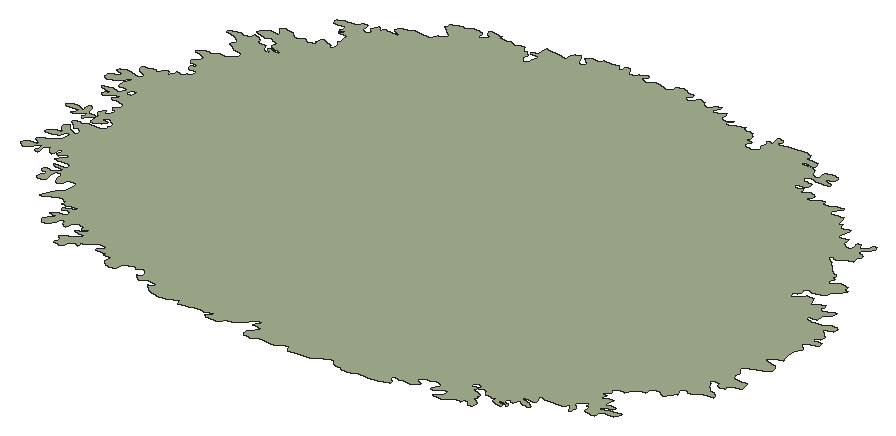
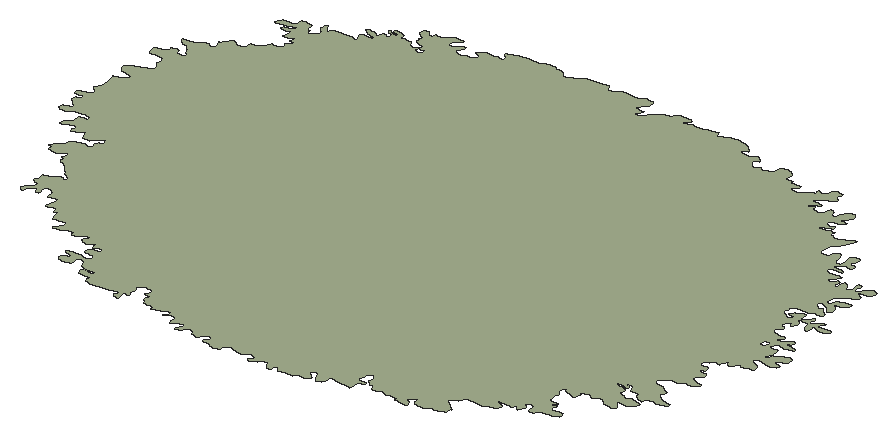
# SketchUp Ruby script. Lengths in inches.
U = 1.inch
M = Sketchup.active_model
def pt(a) = Geom::Point3d.new(a.map { |v| v * U })
def face(e, loops, mat)
  f = e.add_face(loops[0].map { |a| pt(a) })
  loops[1..].each { |l| e.add_face(l.map { |a| pt(a) }).erase! }
  f.material = f.back_material = mat if mat
  f
end
# faces: each face lists its corners as indices into pts; further lists are holes
def faces(e, pts, list, mat = nil) = list.each { |f| face(e, (f[0].is_a?(Array) ? f : [f]).map { |l| l.map { |i| pts[i] } }, mat) }
# xy, xz, yz: faces in a plane at the given z, y or x. An outline is a flat list of corners, or four numbers for a rectangle; further outlines are holes
def ring(l) = l.size == 4 ? [[l[0], l[1]], [l[2], l[1]], [l[2], l[3]], [l[0], l[3]]] : l.each_slice(2).to_a
def flat(e, list, mat, &to3) = list.each { |f| face(e, (f[0].is_a?(Array) ? f : [f]).map { |l| ring(l).map { |u, v| to3.(u, v) } }, mat) }
def xy(e, z, list, mat = nil) = flat(e, list, mat) { |x, y| [x, y, z] }
def xz(e, y, list, mat = nil) = flat(e, list, mat) { |x, z| [x, y, z] }
def yz(e, x, list, mat = nil) = flat(e, list, mat) { |y, z| [x, y, z] }
def lines(e, pts, list) = list.each { |a, b| e.add_line(pt(pts[a]), pt(pts[b])) }
# prism: a flat outline (further loops are holes) pulled along v
def prism(e, loops, v, mat = nil)
  f = face(e, loops, mat); d = Geom::Vector3d.new(v.map { |x| x * U })
  f.pushpull(f.normal.samedirection?(d) ? d.length : -d.length)
end
def box(e, o, s, mat = nil) = prism(e, [[o, [o[0] + s[0], o[1], o[2]], [o[0] + s[0], o[1] + s[1], o[2]], [o[0], o[1] + s[1], o[2]]]], [0, 0, s[2]], mat)
def at(x, y, z, deg = 0) = Geom::Transformation.translation(pt([x, y, z])) * Geom::Transformation.rotation(ORIGIN, Z_AXIS, deg.degrees)
def axes(o, x, y, z) = Geom::Transformation.new([*x, 0, *y, 0, *z, 0, *pt(o).to_a, 1])
def part(name) = M.definitions.add(name)
# library, detail: a bought-in or finely detailed component or shape, given as its bounding box
def library(name, o, s) = part(name).tap { |d| box(d.entities, o, s) }
def detail(e, o, s) = box(e.add_group.entities, o, s)
def put(e, d, t, mat = nil) = e.add_instance(d, t).tap { |i| i.material = mat if mat }
def group(e, t, mat = nil) = e.add_group.tap { |g| g.transformation = t; g.material = mat if mat }.entities
root = M.entities
M.materials.add("Boxwoodplan").color = [166, 177, 144]
xy(root,9.058,[[[105.479,67.129,105.368,67.133,105.273,67.159,105.217,67.215,105.216,67.317,105.242,67.382,105.305,67.445,105.354,67.509,105.413,67.606,105.226,67.635,105.136,67.644,105.156,67.732,105.242,67.79,105.273,67.8,105.268,67.846,105.179,67.877,105.063,67.837,104.966,67.706,104.824,67.551,104.663,67.464,104.557,67.441,104.497,67.416,104.481,67.373,104.336,67.281,104.143,67.251,104.054,67.26,103.973,67.306,103.973,67.328,104.019,67.359,104.109,67.437,104.178,67.483,104.088,67.498,103.976,67.48,103.856,67.436,103.662,67.454,103.565,67.447,103.439,67.403,103.238,67.356,103.149,67.349,103.111,67.443,103.103,67.465,103.036,67.473,102.947,67.454,102.779,67.336,102.579,67.328,102.349,67.353,102.182,67.446,102.04,67.61,102.223,67.702,102.124,67.756,101.988,67.772,101.862,67.749,101.789,67.697,101.709,67.672,101.593,67.738,101.551,67.806,101.638,67.847,101.665,67.907,101.67,67.957,101.629,68.009,101.556,68.085,101.471,68.117,101.384,68.064,101.317,68.038,101.261,68.08,101.245,68.103,101.221,68.121,101.191,68.111,101.112,68.058,101.04,68.01,100.964,67.923,100.953,67.79,100.881,67.749,100.831,67.723,100.771,67.725,100.672,67.746,100.586,67.793,100.542,67.861,100.533,67.951,100.542,68.018,100.555,68.04,100.536,68.08,100.323,68.1,100.391,68.135,100.364,68.136,100.272,68.13,100.102,68.146,100.025,68.173,100.008,68.206,100.022,68.224,100.148,68.314,100.145,68.371,100.061,68.393,99.901,68.39,99.771,68.319,99.673,68.233,99.599,68.199,99.551,68.172,99.55,68.154,99.587,68.101,99.571,68.046,99.5,68.081,99.437,68.121,99.376,68.072,99.353,68.017,99.322,67.904,99.274,67.855,99.201,67.822,99.11,67.816,99.04,67.841,99.022,67.874,99.029,67.892,99.05,67.932,99.072,67.991,99.041,68.048,98.94,68.149,99.054,68.229,99.115,68.269,99.194,68.285,99.262,68.315,99.317,68.37,99.401,68.476,99.33,68.503,99.25,68.511,99.118,68.53,99.079,68.565,99.087,68.584,99.161,68.62,99.323,68.657,99.366,68.709,99.361,68.748,99.335,68.764,99.185,68.711,99.139,68.732,99.14,68.752,99.162,68.814,99.001,68.825,98.921,68.833,98.867,68.826,98.859,68.806,98.843,68.71,98.828,68.642,98.787,68.591,98.74,68.578,98.72,68.594,98.661,68.639,98.617,68.757,98.577,68.783,98.55,68.784,98.497,68.777,98.49,68.757,98.488,68.641,98.433,68.523,98.373,68.449,98.293,68.419,98.214,68.422,98.167,68.448,98.134,68.506,98.135,68.564,98.188,68.677,98.302,68.784,98.323,68.803,98.309,68.823,98.283,68.829,98.202,68.847,98.122,68.86,98.095,68.875,98.101,68.895,98.122,68.914,98.27,68.982,98.432,69.005,98.474,69.108,98.448,69.169,98.401,69.191,98.373,69.187,98.21,69.168,98.17,69.2,98.176,69.22,98.204,69.279,98.361,69.334,98.533,69.403,98.582,69.442,98.568,69.463,98.472,69.436,98.3,69.417,98.156,69.372,98.067,69.386,98.04,69.392,98.047,69.412,98.067,69.426,98.122,69.47,98.095,69.507,98.067,69.503,97.985,69.511,97.93,69.56,97.916,69.601,97.888,69.597,97.806,69.575,97.649,69.489,97.499,69.413,97.425,69.38,97.37,69.392,97.383,69.412,97.403,69.452,97.429,69.469,97.454,69.55,97.503,69.65,97.535,69.759,97.586,69.812,97.66,69.852,97.704,69.972,97.726,70.112,97.745,70.227,97.741,70.285,97.696,70.321,97.616,70.335,97.529,70.335,97.456,70.31,97.446,70.245,97.446,70.184,97.413,70.124,97.325,70.087,97.269,70.096,97.23,70.155,97.22,70.216,97.194,70.337,97.188,70.4,97.148,70.453,97.12,70.475,97.083,70.491,97.024,70.479,96.989,70.46,96.988,70.428,96.98,70.366,96.982,70.229,97.007,70.167,96.999,70.103,96.949,70.038,96.9,70.01,96.862,69.998,96.825,70.003,96.783,70.011,96.765,70.039,96.761,70.166,96.782,70.223,96.827,70.276,96.843,70.306,96.834,70.334,96.777,70.34,96.696,70.346,96.658,70.362,96.635,70.39,96.632,70.453,96.648,70.483,96.682,70.499,96.855,70.472,96.933,70.497,96.983,70.526,97.043,70.573,97.057,70.636,97.034,70.662,96.99,70.664,96.912,70.67,96.82,70.681,96.719,70.717,96.701,70.746,96.706,70.76,96.726,70.763,96.785,70.775,96.961,70.761,97.05,70.787,97.063,70.844,97.037,70.907,96.965,70.946,96.886,70.953,96.772,70.946,96.673,70.921,96.589,70.939,96.585,70.968,96.606,70.997,96.652,71.054,96.719,71.11,96.772,71.19,96.763,71.224,96.719,71.241,96.654,71.24,96.536,71.14,96.496,71.141,96.462,71.161,96.483,71.22,96.5,71.287,96.456,71.35,96.416,71.366,96.396,71.367,96.391,71.352,96.395,71.306,96.392,71.164,96.351,71.102,96.311,71.108,96.277,71.131,96.179,71.262,96.154,71.327,96.13,71.355,96.114,71.344,96.059,71.293,96.024,71.234,96.043,71.103,96.048,71.037,96.028,70.971,95.979,70.962,95.944,70.978,95.934,71.023,95.954,71.155,95.964,71.233,95.964,71.27,95.949,71.282,95.934,71.272,95.854,71.237,95.815,71.183,95.805,71.12,95.766,71.077,95.629,70.987,95.59,70.977,95.545,70.986,95.466,71.026,95.445,71.056,95.449,71.089,95.482,71.151,95.58,71.237,95.669,71.263,95.759,71.263,95.854,71.267,95.794,71.318,95.642,71.404,95.626,71.466,95.679,71.503,95.77,71.573,95.889,71.635,96.008,71.709,96.043,71.723,96.069,71.746,96.096,71.789,96.099,71.882,96.131,72.003,96.132,72.065,96.111,72.086,96.09,72.095,96.027,72.109,95.993,72.104,95.99,72.088,96.001,71.996,95.96,71.934,95.912,71.899,95.834,71.871,95.763,71.858,95.603,71.833,95.568,71.839,95.554,71.853,95.555,71.86,95.563,71.901,95.58,71.947,95.622,71.995,95.692,72.042,95.75,72.063,95.809,72.065,95.847,72.068,95.867,72.075,95.89,72.096,95.886,72.121,95.831,72.151,95.763,72.207,95.731,72.264,95.727,72.331,95.74,72.382,95.793,72.426,95.819,72.432,95.83,72.425,95.849,72.411,95.892,72.35,95.941,72.304,96.07,72.226,96.143,72.192,96.179,72.177,96.199,72.184,96.223,72.206,96.229,72.222,96.241,72.263,96.225,72.32,96.183,72.366,96.15,72.389,96.117,72.401,96.057,72.401,95.983,72.404,95.939,72.446,95.853,72.519,95.795,72.569,95.756,72.617,95.756,72.646,95.78,72.671,95.837,72.698,95.872,72.703,95.913,72.7,95.973,72.679,96.034,72.677,96.07,72.684,96.105,72.726,96.153,72.757,96.213,72.764,96.284,72.764,96.4375,72.771,96.578,72.792,96.61,72.808,96.611,72.826,96.605,72.868,96.594,72.913,96.605,72.957,96.635,73.06,96.621,73.083,96.599,73.097,96.542,73.126,96.488,73.164,96.416,73.192,96.343,73.195,96.292,73.184,96.271,73.17,96.246,73.119,96.251,73.098,96.263,73.093,96.286,73.088,96.437,73.076,96.463,73.071,96.469,73.0625,96.459,73.046,96.42,73.007,96.374,72.964,96.31,72.928,96.248,72.884,96.175,72.849,96.138,72.852,96.119,72.863,96.093,72.9,96.086,72.995,96.069,73.02,96.087,73.034,96.094,73.077,96.088,73.088,96.076,73.088,96.062,73.087,96.036,73.083,96.003,73.076,95.986,73.065,95.905,72.97,95.873,72.915,95.842,72.892,95.819,72.895,95.793,72.916,95.784,72.932,95.778,72.973,95.806,73.057,95.812,73.102,95.803,73.13,95.782,73.137,95.744,73.128,95.724,73.114,95.678,73.064,95.557,72.957,95.52,72.932,95.495,72.927,95.457,72.935,95.445,72.951,95.537,73.057,95.599,73.102,95.613,73.129,95.613,73.145,95.604,73.152,95.592,73.148,95.578,73.143,95.546,73.131,95.463,73.108,95.295,73.089,95.222,73.096,95.175,73.121,95.153,73.149,95.152,73.165,95.169,73.217,95.216,73.264,95.277,73.281,95.347,73.284,95.422,73.266,95.549,73.223,95.635,73.197,95.647,73.201,95.647,73.209,95.646,73.22,95.637,73.239,95.613,73.287,95.611,73.342,95.619,73.407,95.63,73.437,95.648,73.45,95.696,73.413,95.736,73.363,95.763,73.317,95.772,73.255,95.785,73.204,95.799,73.176,95.823,73.175,95.957,73.157,96.03,73.144,96.065,73.14,96.083,73.154,96.099,73.202,96.043,73.244,95.985,73.309,95.967,73.335,95.967,73.352,96.001,73.46,96.031,73.483,96.059,73.489,96.073,73.477,96.082,73.459,96.111,73.414,96.123,73.39,96.135,73.391,96.156,73.404,96.236,73.482,96.252,73.528,96.254,73.579,96.24,73.611,96.219,73.623,96.155,73.646,96.116,73.666,96.107,73.687,96.123,73.736,96.179,73.773,96.214,73.795,96.227,73.816,96.234,73.869,96.233,73.916,96.137,73.992,95.994,74.014,95.931,74.031,95.897,74.013,95.868,74.014,95.799,74.031,95.78,74.058,95.79,74.082,95.916,74.185,95.909,74.217,95.887,74.233,95.843,74.225,95.814,74.216,95.688,74.154,95.648,74.107,95.598,74.063,95.529,74.049,95.501,74.05,95.454,74.102,95.482,74.126,95.5,74.165,95.532,74.188,95.625,74.22,95.67,74.25,95.66,74.281,95.647,74.283,95.637,74.276,95.611,74.27,95.571,74.273,95.436,74.284,95.29,74.3125,95.266,74.327,95.271,74.347,95.296,74.375,95.509,74.435,95.573,74.434,95.633,74.419,95.694,74.391,95.72,74.393,95.727,74.403,95.776,74.48,95.799,74.495,95.806,74.515,95.805,74.557,95.805,74.583,95.795,74.593,95.781,74.591,95.724,74.591,95.666,74.585,95.619,74.568,95.595,74.576,95.575,74.596,95.55,74.63,95.53,74.718,95.54,74.806,95.57,74.848,95.576,74.88,95.589,74.923,95.627,74.944,95.622,74.99,95.6,75.026,95.511,75.003,95.494,74.969,95.495,74.95,95.498,74.886,95.417,74.839,95.276,74.745,95.121,74.7,95.037,74.725,94.995,74.778,94.985,74.904,95.114,74.99,95.196,75.003,95.24,75.027,95.264,75.061,95.262,75.081,95.177,75.112,95.104,75.138,95.042,75.194,95.077,75.249,95.153,75.278,95.249,75.312,95.314,75.311,95.492,75.267,95.585,75.246,95.669,75.25,95.72,75.269,95.726,75.289,95.711,75.355,95.65,75.407,95.605,75.415,95.493,75.485,95.446,75.527,95.431,75.564,95.425,75.617,95.425,75.644,95.4375,75.659,95.48,75.695,95.531,75.709,95.645,75.741,95.675,75.751,95.716,75.75,95.766,75.746,95.778,75.733,95.793,75.703,95.808,75.689,95.817,75.689,95.846,75.692,95.862,75.704,95.882,75.754,95.91,75.787,95.927,75.81,95.929,75.835,95.946,75.86,95.965,75.872,96.013,75.884,96.052,75.877,96.074,75.833,96.078,75.781,96.094,75.755,96.116,75.754,96.157,75.796,96.182,75.838,96.197,75.942,96.212,75.968,96.245,75.975,96.276,75.974,96.296,75.963,96.317,75.94,96.349,75.94,96.401,75.961,96.446,76.007,96.46,76.032,96.449,76.046,96.509,76.043,96.538,76.046,96.553,76.066,96.558,76.114,96.592,76.155,96.627,76.2,96.573,76.243,96.505,76.272,96.468,76.271,96.436,76.261,96.393,76.249,96.352,76.255,96.33,76.271,96.308,76.295,96.285,76.397,96.298,76.423,96.304,76.439,96.314,76.443,96.418,76.463,96.464,76.472,96.483,76.483,96.473,76.486,96.387,76.514,96.321,76.526,96.293,76.519,96.257,76.52,96.221,76.52,96.186,76.532,96.147,76.582,96.129,76.611,96.129,76.642,96.145,76.663,96.174,76.678,96.205,76.697,96.213,76.725,96.243,76.782,96.27,76.836,96.276,76.89,96.268,76.917,96.228,76.928,96.15,76.954,95.977,77.001,95.942,77.018,95.925,77.042,95.96,77.097,96.005,77.131,96.05,77.159,96.105,77.178,96.158,77.1875,96.21,77.184,96.265,77.16,96.321,77.162,96.347,77.167,96.361,77.187,96.378,77.228,96.415,77.264,96.435,77.282,96.462,77.284,96.531,77.267,96.593,77.256,96.619,77.253,96.643,77.268,96.729,77.336,96.817,77.401,96.87,77.498,96.867,77.542,96.825,77.579,96.708,77.617,96.583,77.647,96.496,77.719,96.439,77.755,96.37,77.776,96.342,77.788,96.329,77.808,96.351,77.855,96.399,77.896,96.397,77.981,96.347,78.06,96.217,78.116,95.977,78.196,95.928,78.212,95.908,78.246,95.979,78.31,96.1,78.362,96.206,78.367,96.263,78.353,96.307,78.327,96.355,78.317,96.408,78.326,96.469,78.337,96.499,78.368,96.513,78.448,96.531,78.483,96.584,78.482,96.641,78.471,96.689,78.451,96.756,78.392,96.781,78.358,96.795,78.318,96.796,78.249,96.802,78.245,96.81,78.249,96.837,78.262,96.889,78.268,96.977,78.271,97.057,78.235,97.092,78.17,97.116,78.092,97.186,78.047,97.227,78.035,97.244,78.034,97.271,78.043,97.367,78.05,97.383,78.055,97.363,78.071,97.3,78.095,97.249,78.099,97.21,78.118,97.191,78.152,97.188,78.164,97.192,78.184,97.207,78.191,97.241,78.192,97.283,78.185,97.39,78.156,97.504,78.152,97.556,78.159,97.575,78.162,97.601,78.173,97.557,78.203,97.515,78.213,97.429,78.228,97.371,78.242,97.331,78.244,97.308,78.248,97.283,78.263,97.232,78.289,97.185,78.315,97.162,78.348,97.173,78.404,97.201,78.442,97.242,78.471,97.202,78.502,97.147,78.517,97.105,78.52,97.049,78.528,97.018,78.555,97.001,78.591,96.986,78.6,96.958,78.599,96.842,78.571,96.79,78.557,96.74,78.559,96.693,78.562,96.643,78.578,96.595,78.595,96.555,78.602,96.469,78.65,96.495,78.662,96.496,78.669,96.508,78.709,96.523,78.745,96.549,78.782,96.58,78.814,96.624,78.839,96.677,78.862,96.723,78.873,96.829,78.867,96.906,78.862,96.939,78.858,96.949,78.857,96.949,78.87,96.941,78.912,96.92,78.956,96.884,78.995,96.842,79.026,96.809,79.073,96.811,79.096,96.821,79.117,96.869,79.147,96.921,79.17,96.947,79.169,96.973,79.163,97.028,79.148,97.095,79.142,97.143,79.127,97.166,79.114,97.185,79.095,97.228,79.055,97.267,79.02,97.312,78.989,97.369,78.976,97.422,78.981,97.468,79.01,97.499,79.046,97.548,79.084,97.574,79.083,97.597,79.069,97.637,79.027,97.684,78.994,97.8125,79.019,97.887,79.037,97.928,79.065,97.934,79.085,97.912,79.102,97.861,79.124,97.852,79.147,97.86,79.169,97.875,79.214,97.882,79.273,97.886,79.299,97.909,79.315,97.937,79.316,97.967,79.308,98.009,79.288,98.143,79.248,98.203,79.226,98.243,79.193,98.269,79.153,98.284,79.13,98.291,79.123,98.301,79.126,98.309,79.131,98.341,79.176,98.347,79.212,98.337,79.315,98.316,79.362,98.292,79.397,98.256,79.436,98.246,79.466,98.258,79.477,98.269,79.475,98.29,79.476,98.29,79.484,98.295,79.508,98.287,79.549,98.273,79.705,98.275,79.782,98.159,79.802,98.062,79.804,98,79.8125,97.982,79.819,97.968,79.83,97.981,79.839,98.094,79.882,98.128,79.911,98.128,79.924,98.105,79.948,98.069,79.952,98.016,79.94,97.968,79.918,97.95,79.919,97.935,79.945,97.962,80.028,97.964,80.069,97.964,80.082,97.94,80.103,97.851,80.085,97.738,80.088,97.628,80.105,97.567,80.185,97.565,80.213,97.603,80.25,97.7,80.303,97.748,80.33,97.803,80.335,97.927,80.332,98.019,80.337,98.078,80.346,98.118,80.384,98.159,80.418,98.166,80.461,98.193,80.5,98.248,80.513,98.286,80.509,98.329,80.475,98.34,80.389,98.347,80.3,98.37,80.257,98.426,80.231,98.517,80.212,98.572,80.234,98.59,80.276,98.567,80.319,98.521,80.355,98.464,80.442,98.5,80.521,98.575,80.603,98.594,80.606,98.617,80.576,98.636,80.528,98.711,80.447,98.738,80.421,98.729,80.475,98.711,80.57,98.768,80.587,98.829,80.582,98.956,80.578,99.069,80.575,99.19,80.557,99.209,80.557,99.196,80.587,99.146,80.629,99.015,80.681,98.977,80.689,98.955,80.735,98.957,80.826,98.991,80.871,99.04,80.896,99.156,80.901,99.253,80.91,99.348,80.977,99.475,80.982,99.591,80.971,99.686,80.953,99.807,80.946,99.85,80.991,99.864,81.038,99.907,81.133,99.996,81.187,100.116,81.244,100.127,81.26,100.111,81.294,100.07,81.332,99.963,81.413,99.894,81.487,99.837,81.528,99.78,81.57,99.81,81.577,99.809,81.591,99.805,81.612,99.793,81.679,99.797,81.709,99.832,81.744,99.914,81.785,99.997,81.821,100.036,81.827,100.092,81.826,100.178,81.816,100.202,81.808,100.226,81.81,100.257,81.843,100.309,81.918,100.345,81.932,100.402,81.936,100.504,81.93,100.6,81.898,100.633,81.877,100.662,81.835,100.663,81.765,100.665,81.736,100.67,81.715,100.694,81.704,100.747,81.715,100.792,81.745,100.853,81.798,100.878,81.822,100.9,81.834,100.912,81.85,100.828,81.897,100.79,81.913,100.746,81.956,100.721,82.036,100.722,82.067,100.781,82.083,100.972,82.055,101.069,82.039,101.105,82.026,101.104,81.98,101.114,81.952,101.175,81.948,101.279,81.962,101.38,81.975,101.423,81.971,101.469,81.957,101.497,81.934,101.521,81.933,101.546,81.943,101.69,81.972,101.731,81.981,101.784,81.987,101.82,81.984,101.864,81.957,101.895,81.886,101.921,81.863,101.966,81.844,102.006,81.833,102.046,81.808,102.098,81.753,102.151,81.696,102.138,81.619,102.132,81.545,102.146,81.515,102.177,81.485,102.203,81.461,102.25,81.453,102.287,81.45,102.331,81.481,102.345,81.512,102.346,81.553,102.334,81.628,102.37,81.787,102.359,81.817,102.341,81.829,102.318,81.833,102.279,81.834,102.227,81.828,102.19,81.826,102.144,81.835,102.118,81.858,102.126,81.88,102.153,81.896,102.193,81.91,102.238,81.937,102.263,82.013,102.266,82.178,102.267,82.21,102.289,82.228,102.316,82.233,102.414,82.222,102.613,82.201,102.705,82.19,102.793,82.169,102.88,82.153,102.931,82.147,102.927,82.355,102.995,82.427,103.079,82.486,103.134,82.477,103.161,82.441,103.21,82.37,103.233,82.297,103.241,82.26,103.239,82.241,103.266,82.206,103.371,82.173,103.423,82.173,103.461,82.204,103.464,82.279,103.362,82.36,103.284,82.419,103.296,82.453,103.34,82.49,103.433,82.541,103.483,82.55,103.564,82.538,103.669,82.537,103.691,82.615,103.901,82.643,104.002,82.661,104.109,82.647,104.189,82.578,104.222,82.543,104.248,82.541,104.288,82.568,104.286,82.643,104.278,82.685,104.29,82.72,104.341,82.729,104.396,82.715,104.467,82.621,104.488,82.548,104.521,82.513,104.569,82.498,104.62,82.503,104.667,82.53,104.755,82.613,104.836,82.668,104.9375,82.715,104.986,82.7,104.999,82.663,104.948,82.592,104.922,82.557,104.93,82.515,105.018,82.457,105.118,82.443,105.169,82.452,105.218,82.498,105.297,82.566,105.411,82.581,105.526,82.553,105.558,82.523,105.634,82.492,105.735,82.511,105.816,82.565,105.816,82.678,105.874,82.721,105.987,82.745,106.092,82.74,106.173,82.681,106.319,82.66,106.372,82.651,106.378,82.614,106.305,82.546,106.272,82.473,106.284,82.437,106.355,82.396,106.458,82.401,106.51,82.433,106.53,82.472,106.551,82.544,106.599,82.567,106.623,82.579,106.675,82.579,106.778,82.541,106.821,82.47,106.906,82.417,107.037,82.447,107.071,82.478,107.078,82.52,107.117,82.603,107.224,82.622,107.254,82.592,107.26,82.55,107.208,82.466,107.159,82.448,107.132,82.413,107.193,82.349,107.323,82.337,107.414,82.373,107.482,82.444,107.506,82.45,107.515,82.433,107.534,82.392,107.558,82.357,107.546,82.301,107.527,82.257,107.545,82.222,107.634,82.179,107.742,82.184,107.797,82.203,107.847,82.258,107.864,82.273,107.867,82.255,107.853,82.212,107.781,82.132,107.747,82.102,107.758,82.066,107.805,82.047,107.862,82.048,107.959,82.088,108.041,82.146,108.261,82.225,108.282,82.153,108.305,82.123,108.357,82.118,108.472,82.11,108.596,82.084,108.611,82.013,108.634,81.983,108.681,81.964,108.704,81.93,108.689,81.892,108.663,81.795,108.779,81.773,108.825,81.755,108.836,81.72,108.762,81.65,108.747,81.613,108.764,81.579,108.839,81.527,108.943,81.5,109.044,81.496,109.156,81.563,109.198,81.639,109.14,81.71,109.107,81.779,109.127,81.885,109.136,81.922,109.107,81.956,109.103,81.992,109.144,82.018,109.245,82.022,109.234,82.122,109.193,82.274,109.242,82.287,109.307,82.275,109.36,82.256,109.392,82.199,109.342,82.131,109.345,82.095,109.392,82.076,109.5,82.076,109.629,82.111,110.137,82.178,110.182,82.168,110.228,82.145,110.275,82.121,110.309,82.097,110.34,82.027,110.322,81.935,110.527,81.949,110.592,81.943,110.676,81.911,110.713,81.805,110.699,81.757,110.682,81.724,110.641,81.717,110.472,81.749,110.407,81.755,110.365,81.755,110.344,81.749,110.341,81.733,110.37,81.685,110.41,81.666,110.458,81.666,110.63,81.681,110.699,81.683,110.784,81.648,110.821,81.609,110.851,81.546,110.919,81.437,110.999,81.398,111.083,81.394,111.114,81.435,111.108,81.518,111.09,81.571,111.097,81.637,111.138,81.687,111.24,81.719,111.349,81.732,111.4375,81.701,111.485,81.659,111.519,81.597,111.52,81.551,111.459,81.495,111.392,81.482,111.351,81.471,111.319,81.437,111.323,81.407,111.373,81.389,111.471,81.363,111.542,81.339,111.562,81.306,111.55,81.275,111.496,81.247,111.408,81.24,111.247,81.233,111.159,81.222,111.071,81.256,111.006,81.269,110.925,81.251,110.868,81.208,110.867,81.143,110.925,81.103,111.012,81.081,111.097,81.066,111.144,81.066,111.178,81.046,111.2,81.003,111.183,80.938,111.148,80.89,111.12,80.866,111.075,80.854,110.932,80.834,110.912,80.829,110.903,80.784,110.908,80.751,110.952,80.732,111.02,80.731,111.061,80.731,111.111,80.746,111.174,80.778,111.188,80.712,111.158,80.665,111.152,80.635,111.191,80.617,111.252,80.622,111.333,80.67,111.389,80.711,111.417,80.736,111.455,80.721,111.519,80.704,111.588,80.651,111.584,80.603,111.541,80.537,111.508,80.472,111.527,80.448,111.574,80.445,111.649,80.456,111.731,80.495,111.77,80.554,111.842,80.597,111.902,80.609,111.939,80.601,111.958,80.577,111.961,80.548,111.944,80.521,111.916,80.497,111.918,80.483,111.938,80.481,112.11,80.499,112.191,80.51,112.258,80.552,112.3,80.589,112.379,80.614,112.476,80.619,112.5,80.595,112.503,80.566,112.342,80.349,112.357,80.304,112.414,80.251,112.497,80.237,112.587,80.255,112.655,80.283,112.739,80.305,112.804,80.213,112.841,79.999,112.842,79.985,112.879,79.974,112.962,79.996,112.973,79.918,112.997,79.871,113.073,79.861,113.211,79.896,113.279,79.893,113.293,79.839,113.225,79.619,113.215,79.567,113.238,79.514,113.304,79.486,113.372,79.496,113.508,79.523,113.528,79.419,113.523,79.316,113.645,79.247,113.777,79.216,113.808,79.318,113.797,79.421,113.775,79.474,113.803,79.525,113.871,79.535,113.91,79.482,113.932,79.429,113.98,79.395,114.058,79.418,114.111,79.467,114.136,79.583,114.139,79.636,114.2,79.659,114.258,79.631,114.288,79.577,114.262,79.455,114.147,79.375,114.094,79.339,114.074,79.282,114.054,79.231,114.076,79.186,114.208,79.161,114.265,79.134,114.269,79.083,114.197,78.997,114.231,78.895,114.261,78.844,114.249,78.794,114.115,78.768,114.013,78.729,113.91,78.658,113.858,78.623,113.793,78.626,113.729,78.659,113.696,78.667,113.67,78.643,113.715,78.549,113.834,78.483,113.88,78.445,113.877,78.396,113.962,78.32,114.129,78.132,114.26,78.05,114.324,78.035,114.361,77.992,114.346,77.898,114.461,77.834,114.398,77.749,114.378,77.697,114.377,77.673,114.408,77.661,114.545,77.679,114.68,77.755,114.809,77.768,114.934,77.734,114.938,77.687,114.871,77.66,114.846,77.644,114.86,77.62,114.9375,77.599,115.009,77.596,115.041,77.595,115.055,77.571,114.966,77.482,114.8,77.322,114.776,77.232,114.772,77.187,114.745,77.142,114.651,77.067,114.523,77.038,114.398,77.043,114.29,77.082,114.22,77.076,114.193,77.004,114.221,76.894,114.191,76.787,114.073,76.72,114.101,76.62,114.239,76.642,114.411,76.833,114.639,76.815,114.715,76.605,114.76,76.595,114.841,76.618,114.929,76.723,115.067,76.735,115.104,76.635,115.054,76.574,115.04,76.539,115.116,76.501,115.255,76.531,115.375,76.598,115.422,76.614,115.511,76.592,115.489,76.477,115.379,76.384,115.314,76.289,115.321,76.113,115.307,76.078,115.215,76.056,115.082,76.087,115.107,75.981,115.239,75.941,115.385,75.936,115.533,75.965,115.77,76.087,115.907,76.099,115.999,76.008,115.966,75.905,115.826,75.849,115.778,75.825,115.75,75.766,115.853,75.675,116.004,75.515,115.972,75.414,115.855,75.359,115.819,75.335,115.858,75.274,116.001,75.269,116.132,75.247,116.143,75.145,116.071,75.089,115.937,75.078,115.812,75.041,115.769,74.942,115.9375,74.761,115.83,74.568,115.834,74.388,115.888,74.176,115.932,74.078,115.799,74.051,115.676,74.008,115.583,73.931,115.555,73.869,115.667,73.801,115.918,73.744,115.995,73.662,116.016,73.559,115.974,73.467,115.86,73.394,115.399,73.234,115.4,73.141,115.444,73.048,115.498,72.954,115.5,72.863,115.491,72.773,115.517,72.719,115.638,72.676,115.763,72.672,115.89,72.682,115.931,72.68,115.989,72.633,116,72.453,115.973,72.395,115.864,72.347,115.738,72.33,115.697,72.331,115.65,72.281,115.693,72.191,115.679,72.163,115.595,72.144,115.554,72.145,115.484,72.17,115.451,72.26,115.382,72.292,115.258,72.297,115.216,72.291,115.201,72.233,115.276,72.156,115.363,71.992,115.392,71.969,115.418,71.918,115.435,71.888,115.516,71.877,115.597,71.86,115.682,71.792,115.745,71.71,115.742,71.681,115.657,71.656,115.409,71.616,115.213,71.488,115.14,71.469,115.046,71.544,115.006,71.553,114.942,71.52,114.945,71.435,115.001,71.27,114.959,71.264,114.925,71.219,114.876,71.18,114.823,71.066,114.784,71.019,114.749,71,114.714,71.013,114.591,71.1,114.529,71.115,114.486,71.116,114.441,71.098,114.378,71.063,114.348,70.991,114.357,70.938,114.339,70.874,114.178,70.852,114.125,70.81,114.093,70.759,114.047,70.718,114.035,70.655,114.004,70.609,113.97,70.583,113.932,70.573,113.863,70.564,113.765,70.575,113.705,70.55,113.644,70.502,113.614,70.457,113.688,70.419,113.715,70.376,113.679,70.32,113.625,70.284,113.604,70.225,113.603,70.209,113.601,70.194,113.621,70.186,113.692,70.18,113.718,70.182,113.738,70.182,113.742,70.166,113.705,70.097,113.685,70.049,113.682,70.02,113.723,70.018,113.863,70.094,113.931,70.11,114.013,70.107,113.996,70.004,113.979,69.89,113.979,69.843,114.002,69.82,114.042,69.818,114.105,69.845,114.186,69.846,114.245,69.832,114.285,69.827,114.292,69.798,114.252,69.76,114.173,69.73,114.106,69.722,114.023,69.696,113.984,69.658,113.968,69.602,113.971,69.587,114.011,69.586,114.094,69.611,114.251,69.673,114.406,69.703,114.531,69.705,114.584,69.685,114.559,69.611,114.538,69.569,114.476,69.518,114.324,69.492,114.184,69.491,114.124,69.482,114.093,69.427,114.118,69.308,114.103,69.264,114.022,69.243,113.886,69.255,113.828,69.261,113.784,69.314,113.776,69.426,113.775,69.468,113.763,69.496,113.755,69.511,113.735,69.512,113.676,69.525,113.672,69.581,113.673,69.595,113.67,69.61,113.65,69.614,113.571,69.617,113.513,69.591,113.469,69.536,113.431,69.499,113.407,69.44,113.417,69.391,113.473,69.354,113.548,69.254,113.544,69.155,113.536,69.115,113.528,69.088,113.497,69.066,113.478,69.067,113.456,69.098,113.427,69.157,113.362,69.258,113.321,69.298,113.308,69.312,113.297,69.299,113.29,69.271,113.287,69.227,113.268,69.173,113.262,69.16,113.232,69.144,113.148,69.137,113.008,69.139,112.721,69.14,112.664,69.162,112.577,69.173,112.557,69.163,112.551,69.133,112.602,69.074,112.627,68.976,112.62,68.936,112.589,68.896,112.564,68.889,112.504,68.88,112.401,68.88,112.304,68.884,112.255,68.853,112.311,68.829,112.412,68.814,112.519,68.78,112.594,68.726,112.675,68.654,112.657,68.629,112.597,68.614,112.496,68.621,112.458,68.63,112.408,68.65,112.359,68.684,112.309,68.708,112.274,68.63,112.265,68.558,112.224,68.545,112.168,68.558,112.124,68.589,112.111,68.6,112.092,68.608,112.081,68.59,112.047,68.513,112.048,68.485,112.082,68.448,112.174,68.416,112.212,68.383,112.226,68.34,112.224,68.326,112.204,68.323,112.162,68.36,112.082,68.409,111.988,68.427,111.931,68.429,111.92,68.415,111.941,68.39,112.055,68.347,112.091,68.335,112.115,68.292,112.111,68.264,112.109,68.251,112.066,68.249,111.954,68.26,111.849,68.295,111.814,68.325,111.805,68.371,111.803,68.441,111.753,68.461,111.693,68.442,111.593,68.449,111.495,68.467,111.468,68.489,111.443,68.526,111.447,68.568,111.453,68.583,111.415,68.591,111.321,68.616,111.282,68.618,111.263,68.619,111.228,68.606,111.216,68.577,111.197,68.571,111.17,68.597,111.166,68.612,111.197,68.635,111.212,68.646,111.205,68.671,111.117,68.729,111.08,68.752,111.061,68.756,110.981,68.716,110.961,68.71,110.949,68.681,110.972,68.59,111.068,68.587,111.106,68.582,111.137,68.541,111.13,68.513,111.124,68.499,111.131,68.471,111.243,68.434,111.33,68.396,111.392,68.338,111.408,68.3125,111.407,68.299,111.373,68.283,111.353,68.273,111.384,68.251,111.438,68.225,111.45,68.2,111.4,68.168,111.388,68.141,111.413,68.106,111.498,68.062,111.575,67.994,111.575,67.851,111.553,67.825,111.501,67.814,111.447,67.829,111.41,67.874,111.369,67.939,111.352,67.949,111.314,67.944,111.261,67.926,111.24,67.897,111.241,67.854,111.24,67.84,111.206,67.828,111.03,67.819,111.021,67.826,110.974,67.808,110.93,67.777,110.846,67.692,110.793,67.661,110.72,67.651,110.582,67.643,110.528,67.658,110.525,67.698,110.634,67.762,110.735,67.834,110.732,67.937,110.725,67.98,110.726,67.994,110.694,68.015,110.635,68.034,110.56,68.034,110.477,67.95,110.457,67.911,110.399,67.866,110.385,67.857,110.348,67.865,110.312,67.88,110.299,67.907,110.34,67.999,110.399,68.094,110.401,68.135,110.333,68.189,110.221,68.224,110.17,68.246,110.132,68.238,110.108,68.215,110.074,68.171,110.041,68.156,109.999,68.157,109.943,68.166,109.905,68.168,109.867,68.145,109.787,68.05,109.8,68.01,109.874,67.97,109.929,67.938,109.957,67.917,109.966,67.89,109.942,67.851,109.881,67.807,109.78,67.756,109.724,67.735,109.651,67.738,109.596,67.76,109.523,67.769,109.477,67.745,109.441,67.743,109.409,67.76,109.354,67.766,109.281,67.752,109.258,67.717,109.269,67.659,109.365,67.575,109.393,67.536,109.393,67.497,109.375,67.492,109.086,67.391,108.81,67.369,108.577,67.373,108.487,67.371,108.364,67.31,108.261,67.275,108.164,67.279,108.127,67.281,108.077,67.299,108.029,67.328,107.969,67.325,107.88,67.334,107.796,67.376,107.736,67.433,107.704,67.478,107.646,67.491,107.546,67.479,107.451,67.438,107.37,67.398,107.271,67.325,107.174,67.269,107.081,67.24,106.84,67.222,106.65,67.186,106.554,67.19,106.489,67.284,106.458,67.351,106.369,67.365,106.278,67.352,106.182,67.28,106.117,67.217,106.027,67.21,105.851,67.233,105.665,67.24,105.587,67.189],[95.987,74.415,96.03,74.419,96.049,74.422,96.075,74.431,96.087,74.474,96.088,74.513,96.095,74.597,96.087,74.631,96.075,74.643,96.076,74.658,96.032,74.635,95.976,74.612,95.957,74.606,95.941,74.59,95.919,74.557,95.91,74.52,95.912,74.476,95.931,74.437,95.949,74.421]]],"Boxwoodplan")
